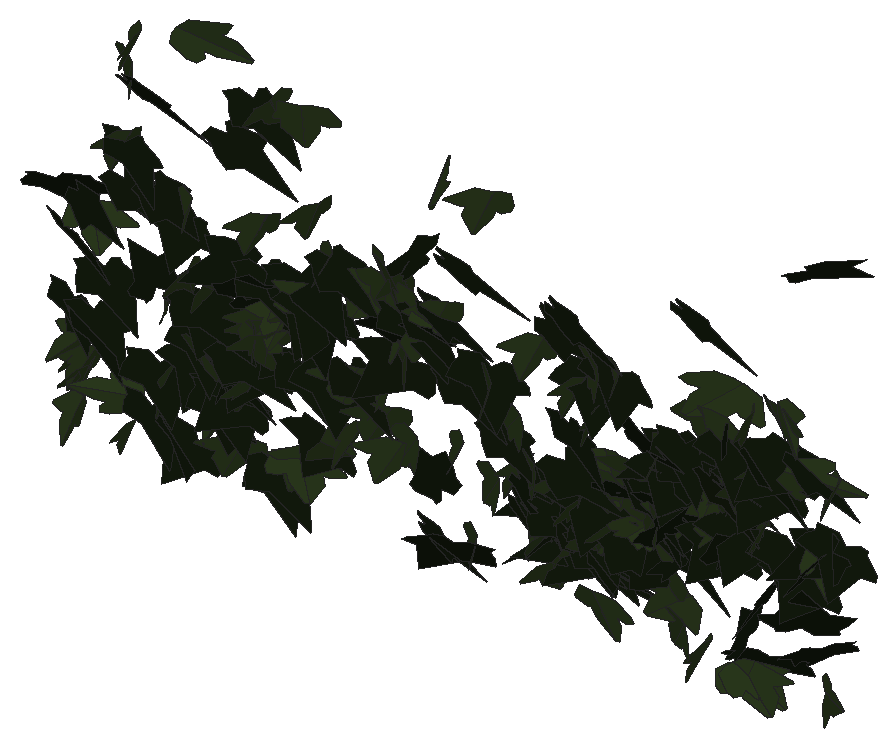
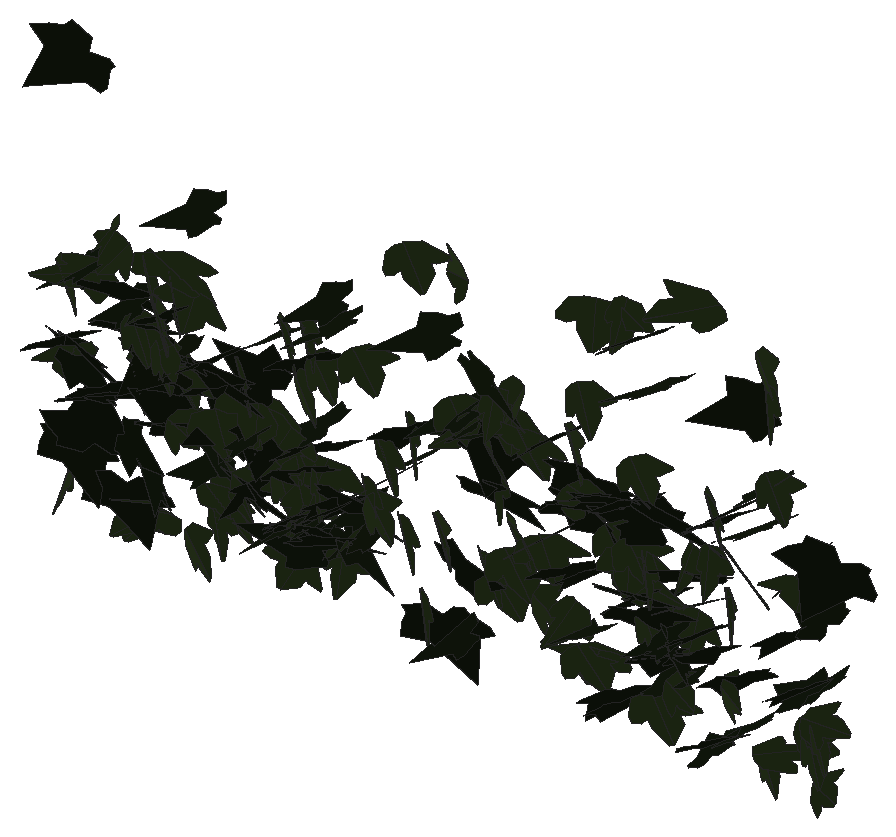
# SketchUp Ruby script. Lengths in millimetres.
U = 1.mm
M = Sketchup.active_model
def pt(a) = Geom::Point3d.new(a.map { |v| v * U })
def face(e, loops, mat)
  f = e.add_face(loops[0].map { |a| pt(a) })
  loops[1..].each { |l| e.add_face(l.map { |a| pt(a) }).erase! }
  f.material = f.back_material = mat if mat
  f
end
# faces: each face lists its corners as indices into pts; further lists are holes
def faces(e, pts, list, mat = nil) = list.each { |f| face(e, (f[0].is_a?(Array) ? f : [f]).map { |l| l.map { |i| pts[i] } }, mat) }
# xy, xz, yz: faces in a plane at the given z, y or x. An outline is a flat list of corners, or four numbers for a rectangle; further outlines are holes
def ring(l) = l.size == 4 ? [[l[0], l[1]], [l[2], l[1]], [l[2], l[3]], [l[0], l[3]]] : l.each_slice(2).to_a
def flat(e, list, mat, &to3) = list.each { |f| face(e, (f[0].is_a?(Array) ? f : [f]).map { |l| ring(l).map { |u, v| to3.(u, v) } }, mat) }
def xy(e, z, list, mat = nil) = flat(e, list, mat) { |x, y| [x, y, z] }
def xz(e, y, list, mat = nil) = flat(e, list, mat) { |x, z| [x, y, z] }
def yz(e, x, list, mat = nil) = flat(e, list, mat) { |y, z| [x, y, z] }
def lines(e, pts, list) = list.each { |a, b| e.add_line(pt(pts[a]), pt(pts[b])) }
# prism: a flat outline (further loops are holes) pulled along v
def prism(e, loops, v, mat = nil)
  f = face(e, loops, mat); d = Geom::Vector3d.new(v.map { |x| x * U })
  f.pushpull(f.normal.samedirection?(d) ? d.length : -d.length)
end
def box(e, o, s, mat = nil) = prism(e, [[o, [o[0] + s[0], o[1], o[2]], [o[0] + s[0], o[1] + s[1], o[2]], [o[0], o[1] + s[1], o[2]]]], [0, 0, s[2]], mat)
def at(x, y, z, deg = 0) = Geom::Transformation.translation(pt([x, y, z])) * Geom::Transformation.rotation(ORIGIN, Z_AXIS, deg.degrees)
def axes(o, x, y, z) = Geom::Transformation.new([*x, 0, *y, 0, *z, 0, *pt(o).to_a, 1])
def part(name) = M.definitions.add(name)
# library, detail: a bought-in or finely detailed component or shape, given as its bounding box
def library(name, o, s) = part(name).tap { |d| box(d.entities, o, s) }
def detail(e, o, s) = box(e.add_group.entities, o, s)
def put(e, d, t, mat = nil) = e.add_instance(d, t).tap { |i| i.material = mat if mat }
def group(e, t, mat = nil) = e.add_group.tap { |g| g.transformation = t; g.material = mat if mat }.entities
root = M.entities
M.materials.add("efeu1").color = [18, 25, 13]
M.materials.add("efeu2").color = [43, 57, 29]
c1 = part("ivyleaf_9")
p = [[39.1,54.8,31.7],[34.5,51.8,30.2],[-5.3,25.2,17.3],[-17.9,28.3,20.9],[-21.6,21.7,17],[-20.2,4.3,5.3],
  [-22.9,-0.3,2.5],[-17.1,-4,-0.6],[-2,-2.1,-1.2],[-0.7,-15.4,-10.1],[16.6,-22.3,-16.7],[21.1,-15.1,-12.5],
  [32.7,-10.7,-11],[46.1,-1.8,-6.6],[30.8,11.2,3.8]]
faces(c1.entities,p,[[0,1,2,3,4,5,6,7,8,9,10,11,12,13,14]],"efeu1")
c2 = part("ivyleaf_10")
p = [[0,12.8,-0.8],[-1.5,51.3,-10.9],[-4.9,51,-11.6],[-13.6,26.5,-7.3],[-13.2,15.9,-4.6],[-21.1,19.3,-7.2],
  [-29.5,16.3,-8.3],[-29.2,8.3,-6.2],[-19.7,-9.8,0.5],[-7.6,-13,4],[1,-12.2,5.8],[-0.4,51.1,-11.1],
  [-1.5,51.1,-10.9],[1,-12.4,5.9],[16.9,-12.4,3.5],[35.1,9.1,-5.1],[35,12.9,-6.1],[20.5,16.4,-4.9],
  [15.8,15,-3.8],[15.3,27.6,-7.1],[12.8,31.3,-7.8]]
faces(c2.entities,p,[[0,1,2,3,4,5,6,7,8,9,10],[11,12,0,13,14,15,16,17,18,19,20]],"efeu2")
put(root,c1,axes([2909.4,930.7,1858.6],[0.80138,-0.79258,-0.01396],[-0.02047,0.01009,-0.89748],[1.50854,0.42118,-0.00476]))
put(root,c1,axes([2143.2,933.4,1731.2],[-0.36983,-0.83025,-0.16051],[0.06105,0.15734,-0.85268],[1.60824,-0.1969,-0.00454]))
put(root,c1,axes([2156,908.4,1846.5],[-0.13639,0.4951,0.78388],[-0.38543,0.75888,-0.49782],[-1.72193,-0.20908,0.04934]))
put(root,c1,axes([2701.6,923.8,1996.9],[1.22093,-0.62842,-0.20152],[-0.109,0.22697,-0.89009],[1.25125,0.63296,0.1191]))
put(root,c1,axes([2747.7,937.1,1774.9],[-0.90081,-0.7438,0.00341],[-0.01004,-0.00068,-0.88162],[1.41559,-0.47333,-0.00408]))
put(root,c2,axes([2666.3,932.6,1941.3],[-0.66779,-0.78909,0.29764],[0.01925,-0.32629,-0.85311],[1.60496,-0.32441,0.13407]))
put(root,c1,axes([2267.2,916.4,1866.7],[0.4535,-0.06865,0.85647],[1.60668,0.18414,-0.22011],[-0.30437,0.86972,0.11421]))
put(root,c1,axes([2043.4,937.4,1745.9],[0.36348,-0.80234,0.30186],[0.21819,-0.28258,-0.82362],[1.61686,0.21851,0.04329]))
put(root,c2,axes([2309.2,917,2120.4],[-0.45151,-0.75455,-0.51758],[0.27982,0.49632,-0.79094],[1.71882,-0.27901,-0.0072]))
put(root,c1,axes([2255.4,923.3,1792.4],[0.4278,-0.6736,-0.50792],[0.182,0.54259,-0.67727],[1.59526,0.11874,0.21347]))
put(root,c1,axes([2503.9,931.8,1918.7],[0.6009,-0.84954,-0.04702],[0.07782,0.06525,-0.90426],[1.61744,0.31248,0.06097]))
put(root,c1,axes([2250.8,943,1722.3],[-1.09629,-0.52426,0.42323],[-0.25126,-0.4582,-0.74726],[1.25746,-0.54862,0.21967]))
put(root,c2,axes([2872.1,917.9,1669.4],[0.99405,-0.52607,-0.47161],[-0.15801,0.53672,-0.69065],[1.33533,0.45513,0.26935]))
put(root,c2,axes([2022.3,939.5,1637.2],[-0.10316,-0.63522,0.62819],[0.45465,-0.61674,-0.60302],[1.63837,0.13115,0.20689]))
put(root,c2,axes([2722.9,931.1,1913.7],[-0.16016,-0.88315,0.16431],[0.02444,-0.16619,-0.88671],[1.70948,-0.08036,0.02807]))
put(root,c1,axes([2127.9,938.4,1670.3],[0.03405,-0.85159,0.1942],[0.09251,-0.19296,-0.85067],[1.65978,0.02823,0.04343]))
put(root,c1,axes([2553.4,922.1,2006.6],[1.44064,-0.53989,-0.11564],[0.11771,0.27791,-0.89262],[1.0442,0.71353,0.26017]))
put(root,c1,axes([2170,941.6,1917.7],[-0.56197,-0.79681,0.27658],[-0.09246,-0.27649,-0.84841],[1.60259,-0.29537,0.04804]))
put(root,c1,axes([2686.8,925.7,1713.1],[-0.77621,0.68802,-0.30967],[0.24728,-0.28272,-0.79924],[-1.41451,-0.42697,0.03022]))
put(root,c1,axes([2492.9,937.6,1909.7],[-0.19363,-0.89325,0.00332],[0.6064,-0.03941,-0.83975],[1.58822,-0.09385,0.32103]))
put(root,c2,axes([2747.6,919.2,1734.6],[-0.66331,-0.67984,-0.44514],[0.39491,0.39384,-0.76396],[1.49528,-0.40559,0.0043]))
put(root,c2,axes([2296.2,924.1,1821.2],[-0.83165,-0.74668,-0.15234],[0.10766,0.14334,-0.86483],[1.44635,-0.44001,-0.02322]))
put(root,c1,axes([2694.6,926,1751.5],[0.13518,-0.72276,-0.49697],[0.06829,0.50057,-0.72287],[1.66795,0.03808,0.06987]))
put(root,c1,axes([3014.2,938.6,1913.5],[-1.56511,-0.36882,0.08779],[-0.06886,-0.13238,-0.89508],[0.71826,-0.81636,0.10548]))
put(root,c2,axes([2959.5,922.8,1639.8],[1.267,0.44384,0.35574],[0.53951,0.21589,-0.79985],[-0.93854,0.72327,0.02045]))
put(root,c2,axes([2269.5,928,1755.5],[-0.18091,-0.87217,-0.01301],[0.0017,0.01299,-0.87734],[1.6601,-0.09506,-0.00052]))
put(root,c1,axes([2207,930.3,1834.1],[-0.0734,-0.75829,-0.43226],[0.70025,0.37823,-0.69635],[1.50639,-0.21277,0.30264]))
put(root,c2,axes([2109.7,928.9,2128.3],[0.40809,-0.89774,-0.02066],[-0.00191,0.021,-0.92299],[1.70904,0.21439,0.0039]))
put(root,c2,axes([2695.2,920.7,1682.6],[-0.56416,-0.76683,-0.36816],[0.1952,0.35481,-0.8216],[1.60711,-0.31229,-0.02945]))
put(root,c1,axes([2950.7,939.7,1806.1],[-0.92835,-0.73922,0.07842],[-0.05571,-0.07463,-0.8855],[1.41369,-0.48838,0.01661]))
put(root,c1,axes([2770.7,942.2,1936],[-0.37873,-0.81888,0.29676],[0.06274,-0.31127,-0.83681],[1.65649,-0.17544,0.09955]))
put(root,c2,axes([2340.9,926.4,1685.7],[1.41976,0.41479,0.1404],[0.24538,0.05701,-0.85346],[-0.79648,0.75694,-0.01266]))
put(root,c1,axes([2246,926.3,2053.1],[0.78076,-0.76261,-0.33412],[0.17649,0.41201,-0.82653],[1.57472,0.33193,0.25829]))
put(root,c2,axes([2750.6,918.6,1947],[0.80962,-0.58843,-0.54919],[-0.23291,0.56667,-0.70195],[1.51407,0.40182,0.18569]))
put(root,c1,axes([2559.2,929.8,1865.2],[0.51469,-0.83253,-0.26467],[0.019,0.27999,-0.87051],[1.6625,0.25454,0.09189]))
put(root,c1,axes([2714.9,924.2,1814.2],[0.52598,-0.69901,-0.55122],[0.25405,0.60319,-0.69798],[1.67508,0.12801,0.27895]))
put(root,c1,axes([2850.7,908.1,1790.6],[-0.16075,0.36952,-0.82506],[-0.3573,0.80342,0.37904],[1.68304,0.20585,0.00167]))
put(root,c2,axes([2354.5,937.7,1885.2],[-0.82762,-0.4296,0.66141],[-0.64951,-0.57841,-0.60007],[1.3532,-0.54037,0.11649]))
put(root,c1,axes([3035.3,925.3,1929.4],[1.00991,-0.66287,-0.33758],[-0.18304,0.35005,-0.83854],[1.40387,0.52249,0.13352]))
put(root,c1,axes([2113.7,926.1,2070.3],[1.58521,-0.35872,0.14303],[0.24879,-0.05806,-0.90688],[0.6916,0.84311,-0.0016]))
put(root,c2,axes([2755.6,926.8,1657.6],[-1.45213,0.31812,-0.17894],[0.26229,-0.13286,-0.82385],[-0.64324,-0.77235,0.06802]))
put(root,c2,axes([2209.7,923.6,1775.3],[-1.48837,0.35112,0.08435],[-0.14945,0.03103,-0.85723],[-0.67081,-0.78596,0.00384]))
put(root,c1,axes([2237.4,935.1,1727.4],[-0.41639,-0.82495,-0.24624],[0.16874,0.23112,-0.85309],[1.62977,-0.2347,0.02541]))
put(root,c1,axes([2983.2,941.7,1876.2],[-1.30263,-0.58294,0.0227],[0.18862,-0.15067,-0.88107],[1.09416,-0.66804,0.1789]))
put(root,c2,axes([2867.7,925.6,1699],[1.32937,-0.30919,-0.4814],[-0.77172,0.26845,-0.76076],[0.76821,0.80472,0.06882]))
put(root,c1,axes([2276.3,932.1,2105.3],[0.27047,-0.86458,-0.27161],[0.16946,0.28692,-0.86673],[1.71641,0.10791,0.12837]))
put(root,c2,axes([2830.2,921.3,1791],[0.86804,-0.62,-0.44837],[-0.1241,0.4886,-0.74194],[1.45091,0.41272,0.20479]))
put(root,c2,axes([2603.8,919,1873.5],[0.58707,-0.76378,-0.61823],[-0.1577,0.62545,-0.81405],[1.86349,0.29355,0.12587]))
put(root,c1,axes([2012.9,941.7,1847.6],[0.3961,-0.66904,0.55304],[0.4288,-0.50759,-0.69884],[1.59541,0.30253,0.05052]))
put(root,c2,axes([2040.7,937.9,1706.9],[-0.2349,-0.76625,0.4123],[0.06756,-0.42052,-0.77089],[1.65466,-0.09161,0.09001]))
put(root,c2,axes([2720.9,925.6,1783.2],[-1.54855,-0.32982,-0.16392],[0.29727,0.05098,-0.87789],[0.63481,-0.82843,0.01124]))
put(root,c1,axes([2363.9,946.7,1708.3],[-0.78177,-0.60773,0.49349],[0.00071,-0.55744,-0.68619],[1.48993,-0.31861,0.25926]))
put(root,c1,axes([2805.4,920.5,1810.1],[1.29284,0.37606,-0.39581],[-0.70484,-0.14687,-0.77512],[-0.7635,0.77236,0.04533]))
put(root,c2,axes([2772.5,930,1752.5],[-0.17268,-0.85028,-0.01671],[0.00166,0.01671,-0.85511],[1.61857,-0.09073,-0.0009]))
put(root,c1,axes([2716.3,935.4,1727.3],[0.50332,-0.84439,-0.0439],[-0.03054,0.04097,-0.88483],[1.60893,0.26493,-0.00307]))
put(root,c2,axes([2726,923.5,1770.5],[-0.08377,-0.80556,-0.36166],[0.05612,0.36057,-0.80672],[1.67963,-0.05222,0.00892]))
put(root,c1,axes([2554.1,925,1657.2],[0.60631,0.61112,-0.55909],[-0.65256,-0.44798,-0.68505],[-1.43498,0.46193,0.0753]))
put(root,c2,axes([2596.1,933.9,2096.5],[-0.89565,-0.75334,0.21424],[-0.01311,-0.24595,-0.87997],[1.49056,-0.45483,0.12099]))
put(root,c1,axes([2363.7,942.7,1877.3],[-0.82308,-0.77497,0.13157],[-0.06355,-0.13192,-0.88679],[1.49467,-0.43236,0.03475]))
put(root,c2,axes([2359.7,929.2,2003.6],[-0.39285,-0.8997,-0.06173],[0.0093,0.06221,-0.92303],[1.71631,-0.20627,-0.00913]))
put(root,c2,axes([3011.8,927.5,1977.9],[-0.23118,0.88578,-0.09809],[0.01783,-0.09773,-0.89406],[-1.69602,-0.12177,0.00397]))
put(root,c1,axes([2289.6,932.8,1897.5],[0.06645,-0.84123,-0.33092],[0.11707,0.33261,-0.83904],[1.71646,0.00988,0.07004]))
put(root,c1,axes([2935.6,941.8,1904.6],[-0.48997,-0.84777,0.09368],[-0.02279,-0.09425,-0.88586],[1.62314,-0.25724,0.01584]))
put(root,c1,axes([2266.9,933.5,1896],[-1.6209,0.1504,0.18177],[-0.35197,-0.00282,-0.86417],[-0.27879,-0.87085,0.03419]))
put(root,c1,axes([2649.2,929.9,1762.8],[1.00563,-0.68049,-0.18562],[-0.16357,0.16808,-0.86085],[1.33241,0.53423,0.03441]))
put(root,c1,axes([2039.4,924.9,1911.3],[0.77836,-0.59364,-0.51117],[-0.50905,0.43617,-0.72054],[1.40136,0.48817,0.02218]))
put(root,c2,axes([2675.8,912,1714],[-0.06921,-0.1733,-0.89781],[0.33355,0.88054,-0.17706],[1.70798,-0.17898,-0.0018]))
put(root,c2,axes([2454.8,925.6,1970.3],[-0.88293,0.76914,-0.00582],[0.00547,-0.00506,-0.89822],[-1.46385,-0.46393,0.00015]))
put(root,c1,axes([2596,939.1,1882.7],[-0.45632,-0.85714,-0.10271],[0.04066,0.10067,-0.89002],[1.64248,-0.24063,-0.0065]))
put(root,c1,axes([2969.3,933.6,1902.3],[0.90871,-0.77371,-0.06069],[-0.0604,0.05174,-0.90917],[1.47581,0.47852,0.00016]))
put(root,c1,axes([2481.1,919.9,1904],[1.26064,0.53861,-0.27147],[-0.46438,-0.12946,-0.8522],[-1.0498,0.70405,0.05098]))
put(root,c1,axes([2351.3,937.1,1866.1],[-0.95766,-0.15655,-0.70433],[1.35564,0.02913,-0.51535],[0.21895,-0.86512,0.1101]))
put(root,c1,axes([3069.9,932.9,1823.1],[-1.59614,0.2784,-0.06454],[0.11299,-0.026,-0.88364],[-0.53203,-0.84074,0.00596]))
put(root,c1,axes([2385.5,930.4,1946.5],[0.4956,-0.79471,-0.38438],[-0.04016,0.39504,-0.83104],[1.67965,0.24394,0.09355]))
put(root,c1,axes([3059.3,933.9,1812.7],[-0.62235,0.59599,-0.5634],[0.48888,-0.50159,-0.67969],[-1.48235,-0.41565,0.01238]))
put(root,c1,axes([2015.2,944.1,1763.8],[0.10234,-0.80925,0.34041],[0.01368,-0.34063,-0.81091],[1.67083,0.05236,-0.01421]))
put(root,c1,axes([2222.6,946.5,1697.2],[-0.32614,-0.69715,0.48712],[0.21817,-0.51131,-0.69145],[1.60385,-0.07221,0.19311]))
put(root,c1,axes([2782.8,942.6,1871.4],[0.51669,-0.43402,0.79329],[0.71368,-0.69966,-0.51113],[1.56604,0.46205,-0.0288]))
put(root,c2,axes([2284.7,935.3,1841.7],[-0.67203,-0.7704,0.22773],[-0.08917,-0.22858,-0.84594],[1.52634,-0.35255,0.05085]))
put(root,c2,axes([2959.1,929.9,1953.9],[0.34956,-0.89419,-0.13502],[0.10629,0.14873,-0.90901],[1.71784,0.17275,0.08372]))
put(root,c1,axes([2870.2,926.7,1753.7],[-0.99186,0.71131,-0.10396],[0.13554,-0.07669,-0.88171],[-1.36142,-0.52586,-0.01204]))
put(root,c2,axes([2309.1,940.4,1854.6],[-0.69625,-0.70571,0.40923],[0.19495,-0.48469,-0.74425],[1.5403,-0.25765,0.27918]))
put(root,c2,axes([2771.8,928.9,1939.7],[0.69799,-0.81694,-0.21878],[-0.05025,0.22729,-0.89297],[1.60881,0.36153,0.06703]))
put(root,c1,axes([2851.7,944.2,1844],[-0.89488,-0.7567,0.0819],[0.05324,-0.11339,-0.88699],[1.44759,-0.46361,0.08325]))
put(root,c2,axes([2349.7,938,1687.2],[-0.88657,-0.6684,0.35346],[-0.15331,-0.36892,-0.80381],[1.43083,-0.45369,0.13288]))
put(root,c2,axes([2960,922.4,1641.9],[0.85557,0.52465,0.53791],[0.63232,0.42344,-0.69066],[-1.28269,0.55869,0.01832]))
put(root,c2,axes([3074.6,932.9,1907.2],[0.5494,-0.86911,-0.03695],[0.03219,0.04453,-0.9153],[1.65527,0.2876,0.03006]))
put(root,c1,axes([3027.9,936.7,1716.6],[1.38149,0.26863,0.52476],[-0.94813,-0.16555,0.77385],[0.5999,-0.88026,0.0146]))
put(root,c1,axes([2339.4,935.3,1909],[-0.61989,-0.45171,-0.70705],[1.22047,0.35507,-0.52225],[1.02972,-0.69277,0.19335]))
put(root,c2,axes([2147.8,942.8,1714.4],[0.38581,-0.66288,0.53641],[0.43104,-0.48971,-0.69076],[1.56463,0.29836,0.05803]))
put(root,c1,axes([2703.2,941.1,1848.1],[0.50053,-0.84001,0.1609],[0.07772,-0.15581,-0.88019],[1.62592,0.26604,-0.00746]))
put(root,c2,axes([2103.1,932.5,1644.1],[0.08856,-0.83337,-0.04496],[0.02224,0.04568,-0.83454],[1.58821,0.04583,0.01419]))
put(root,c1,axes([3033,947.1,1772.6],[-0.95688,-0.65718,0.26594],[-0.06454,-0.30336,-0.81377],[1.34773,-0.48112,0.14984]))
put(root,c2,axes([2461.4,930.4,1942.9],[-1.65897,0.19635,0.09667],[-0.24212,-0.13155,-0.8799],[-0.33893,-0.86709,0.15539]))
put(root,c1,axes([2614.8,934.1,1815.8],[0.47759,-0.8063,-0.26613],[-0.03176,0.27278,-0.84216],[1.61567,0.24371,0.06212]))
put(root,c2,axes([2341.6,930.5,2115.6],[-1.48048,-0.48788,-0.031],[0.08305,-0.01127,-0.91764],[0.92668,-0.77842,0.03272]))
put(root,c1,axes([2094,942,1985.4],[0.18452,-0.88731,0.07237],[0.02041,-0.07163,-0.89259],[1.69421,0.0975,0.00287]))
put(root,c2,axes([2804.7,938.9,1757.1],[0.78708,0.45844,-0.60027],[-0.91223,-0.36961,-0.6125],[-1.11096,0.62828,0.07767]))
put(root,c2,axes([3036.9,923,1913.5],[-0.50836,-0.16322,-0.85574],[1.50202,0.33366,-0.30999],[0.70205,-0.83205,0.04356]))
put(root,c1,axes([3078.9,946.4,1826.1],[-0.65041,-0.79021,0.20626],[-0.07931,-0.20643,-0.85989],[1.55228,-0.34164,0.04249]))
put(root,c2,axes([2780.2,929,1801.5],[-1.45672,0.19796,0.42981],[-0.84965,-0.03105,-0.78071],[-0.29863,-0.87728,0.12462]))
put(root,c2,axes([2898.4,932,1933.2],[-1.64281,0.17521,-0.08906],[0.10143,-0.17745,-0.86567],[-0.36004,-0.84943,0.16247]))
put(root,c1,axes([2339.2,937.7,1796.3],[0.09733,-0.86786,-0.22976],[0.07028,0.23197,-0.86799],[1.70717,0.03993,0.04883]))
put(root,c1,axes([2180.6,947.8,1641.5],[-0.82843,-0.6341,0.34252],[-0.21528,-0.33508,-0.76407],[1.35463,-0.44104,0.08805]))
put(root,c1,axes([2708.5,937.3,1762.5],[-1.62926,0.07646,0.18632],[-0.35471,0.00756,-0.85943],[-0.14525,-0.87607,0.00884]))
put(root,c2,axes([2579.2,927.9,1670.2],[0.63774,-0.71241,-0.32832],[0.00526,0.35809,-0.77419],[1.49292,0.30307,0.14298]))
put(root,c2,axes([2297.2,930.3,1801.9],[-0.12904,-0.01497,0.88164],[-1.6756,-0.04782,-0.06852],[0.09293,-0.88295,-0.01123]))
put(root,c2,axes([2024.8,947.5,1722.4],[-0.18523,-0.42905,0.75789],[-0.04277,-0.76111,-0.43377],[1.65696,-0.06761,0.07353]))
put(root,c2,axes([2607.7,926.6,1752.3],[0.83684,-0.68279,-0.43084],[-0.16965,0.44654,-0.79864],[1.52717,0.42375,0.14737]))
put(root,c2,axes([2404.1,943.7,1736.4],[0.11032,-0.74159,0.49205],[0.14471,-0.48717,-0.74318],[1.68762,0.09025,0.03156]))
put(root,c2,axes([2374,929.7,1945.9],[0.42207,-0.84703,-0.28223],[-0.08251,0.28025,-0.87514],[1.69719,0.22427,0.02764]))
put(root,c1,axes([2923.4,947.4,1776.6],[-1.3141,-0.50333,0.18217],[-0.02029,-0.28433,-0.82602],[1.01855,-0.65505,0.21857]))
put(root,c1,axes([2356.5,945.3,1872.3],[-1.09054,-0.68403,0.03057],[0.05223,-0.06278,-0.89021],[1.3021,-0.57038,0.06132]))
put(root,c1,axes([2738.3,944.3,1920],[-0.58818,-0.83537,0.01129],[0.00024,-0.01208,-0.8907],[1.59002,-0.30902,0.00431]))
put(root,c2,axes([2741.4,936.9,1883.6],[0.41414,-0.87161,0.09066],[0.08772,-0.0819,-0.89803],[1.6655,0.22105,0.02475]))
put(root,c1,axes([2687.9,925.9,1978.5],[1.11091,-0.50997,-0.4535],[-0.23377,0.5085,-0.72992],[1.27762,0.53647,0.26077]))
put(root,c2,axes([2476.8,938.9,1895.4],[0.81879,-0.77724,0.17532],[0.15059,-0.15658,-0.88834],[1.50892,0.43738,-0.00648]))
put(root,c1,axes([2970.2,914.9,1694.7],[-0.60436,0.22971,-0.89619],[-1.32211,0.56659,0.39137],[1.16291,0.76353,-0.0208]))
put(root,c1,axes([2193.2,947.2,1747.8],[-0.69019,-0.7536,0.205],[-0.15741,-0.18769,-0.83629],[1.47801,-0.3719,0.00666]))
put(root,c2,axes([2832.1,928.3,1868.6],[0.46629,-0.76909,-0.39565],[-0.15672,0.38861,-0.8064],[1.63859,0.25603,0.03547]))
put(root,c2,axes([2198.8,920.6,2164.6],[0.73658,0.19598,0.82773],[0.90895,0.70244,-0.38963],[-1.33963,0.58437,0.19075]))
put(root,c1,axes([2483.1,941.6,1850.8],[-1.68287,-0.15992,-0.0197],[0.0401,-0.00578,-0.89853],[0.30404,-0.88443,0.00944]))
put(root,c2,axes([2534.2,921.5,2081.9],[0.65247,-0.52953,0.67862],[-0.5407,0.61992,0.62725],[-1.54641,-0.44017,0.06701]))
put(root,c2,axes([2184.7,926.3,1862.7],[-0.18925,-0.77324,-0.46271],[0.1446,0.45667,-0.77947],[1.70889,-0.12427,0.01472]))
put(root,c2,axes([2973.4,934,1819.7],[0.44374,-0.83809,-0.10634],[0.05389,0.118,-0.86795],[1.60693,0.22747,0.05847]))
put(root,c2,axes([2857.7,925.7,1727.3],[-0.83566,0.34645,0.68714],[-1.26001,0.23321,-0.54063],[-0.74657,-0.78139,0.1433]))
put(root,c1,axes([2870.8,933.2,2051.3],[1.25791,-0.63081,-0.07012],[0.11514,0.1634,-0.89963],[1.20246,0.64426,0.1595]))
put(root,c1,axes([2927.7,920.9,1773],[0.01873,-0.18546,0.87666],[1.21982,0.61414,0.12273],[-1.19179,0.62567,0.13939]))
put(root,c2,axes([2465.5,940.2,1736.6],[-0.97686,-0.62942,0.32203],[-0.16458,-0.33906,-0.80055],[1.33549,-0.50218,0.13689]))
put(root,c1,axes([2861.1,944.9,1878.3],[-0.15904,-0.87928,0.04149],[-0.01195,-0.04108,-0.88324],[1.67526,-0.08377,-0.00236]))
put(root,c1,axes([2740,935.6,1723.1],[0.34268,-0.78707,-0.35039],[0.05645,0.36341,-0.80108],[1.63871,0.15207,0.10087]))
put(root,c1,axes([2990,928,1668.7],[0.70214,0.61662,-0.44663],[-0.62687,-0.31821,-0.71138],[-1.30645,0.48408,0.1013]))
put(root,c2,axes([2809.2,931,1834.2],[-1.79618,-0.01712,0.07843],[-0.14922,-0.00235,-0.94392],[0.03284,-0.94702,0.00092]))
put(root,c1,axes([2404.4,938,1813.9],[0.38693,-0.84803,-0.23704],[-0.01855,0.24109,-0.87089],[1.67573,0.19848,0.04509]))
put(root,c2,axes([2380.8,921.1,1723.9],[-0.40472,-0.59928,-0.74567],[0.54049,0.68989,-0.63544],[1.7386,-0.35397,0.02396]))
put(root,c2,axes([3072,924.1,1652],[0.42654,-0.63918,-0.5683],[0.32212,0.60901,-0.61823],[1.5956,0.04792,0.27672]))
put(root,c2,axes([2510.2,918.4,1909.9],[-0.08743,-0.42333,-0.93647],[1.00073,0.79574,-0.38551],[1.68055,-0.49587,0.18084]))
put(root,c1,axes([2228,942.2,1746.2],[-0.96248,0.29814,-0.64144],[0.97404,-0.39007,-0.58481],[-0.92926,-0.71766,0.05139]))
put(root,c2,axes([2527,940,1932.4],[-0.69637,-0.79289,0.22799],[-0.00369,-0.24858,-0.8676],[1.57017,-0.35223,0.09907]))
put(root,c2,axes([2634.1,928.6,1840.6],[0.97752,-0.58172,-0.4366],[-0.26333,0.44658,-0.75779],[1.359,0.50497,0.16721]))
put(root,c1,axes([2297.7,941.7,1648.8],[-0.11026,-0.83191,-0.14877],[0.00206,0.14905,-0.83388],[1.60841,-0.05722,-0.00913]))
put(root,c2,axes([2554.6,931.7,1774.7],[0.49636,-0.79449,-0.28458],[-0.11436,0.27962,-0.83571],[1.60207,0.26611,0.02851]))
put(root,c1,axes([3056.3,915.9,2176.2],[1.13549,0.59328,0.51411],[0.61219,0.40429,-0.83984],[-1.36291,0.67588,0.05108]))
put(root,c1,axes([2741.6,945.4,1728],[-0.05145,-0.87017,0.04415],[0.0214,-0.04452,-0.8705],[1.65811,-0.02642,0.0126]))
put(root,c2,axes([2856.3,938.4,1800.8],[-1.19006,-0.61241,0.15654],[-0.03419,-0.20289,-0.86548],[1.20253,-0.61183,0.13031]))
put(root,c2,axes([2888.7,940.5,1641.4],[0.26769,-0.87751,0.16074],[0.04352,-0.15913,-0.88871],[1.69732,0.14248,-0.00256]))
put(root,c1,axes([2642.3,931,1737.9],[1.09724,-0.53226,-0.37239],[-0.37722,0.33003,-0.77856],[1.17736,0.60178,0.09761]))
put(root,c1,axes([2792.9,931.3,1743.5],[0.25933,-0.66652,-0.62668],[-0.14641,0.623,-0.67933],[1.735,0.1522,0.03634]))
put(root,c1,axes([2739.6,944.7,1707.9],[-1.51435,-0.29816,0.05171],[-0.08713,-0.02519,-0.84968],[0.56931,-0.79697,0.00751]))
put(root,c1,axes([2978,943.9,1740.5],[-0.64384,0.38007,-0.70218],[0.77581,-0.57352,-0.50682],[-1.30663,-0.5278,0.04508]))
put(root,c2,axes([3060.5,935.8,1814.6],[0.78938,0.7663,-0.07857],[-0.05013,-0.07508,-0.87126],[-1.46521,0.41541,-0.01252]))
put(root,c2,axes([2272.5,926.7,1823.6],[0.73378,-0.60356,-0.56134],[-0.13847,0.59238,-0.68691],[1.56259,0.33592,0.20273]))
put(root,c1,axes([2695.8,948.1,1749.2],[-0.1858,-0.87575,0.11259],[-0.01177,-0.11259,-0.88115],[1.68041,-0.09762,0.00628]))
put(root,c2,axes([2655.2,929.9,1784.5],[0.83717,-0.64748,-0.40782],[-0.08599,0.4476,-0.75937],[1.4538,0.39933,0.18992]))
put(root,c2,axes([2752.3,940.6,1823.9],[1.34766,-0.28038,0.42554],[0.79417,-0.09916,-0.7597],[0.55673,0.82016,0.05362]))
put(root,c2,axes([2934.3,936.4,1857.4],[-0.10947,-0.87897,-0.07927],[0.04312,0.07794,-0.88067],[1.67909,-0.05931,0.01745]))
put(root,c2,axes([2444,939.7,1809.8],[0.91875,-0.73974,0.02869],[0.03221,-0.02322,-0.88332],[1.40857,0.48304,0.00148]))
put(root,c1,axes([2721.9,949.7,1703],[-1.24848,-0.24274,0.48225],[-0.72724,-0.32739,-0.68456],[0.72592,-0.74546,0.14361]))
put(root,c1,axes([2300.8,939.2,1659.7],[-0.05877,-0.80519,-0.39924],[0.05208,0.39845,-0.80571],[1.70968,-0.03982,0.01082]))
put(root,c2,axes([2927.3,939.1,1972.4],[1.55638,0.15887,-0.54508],[-1.04152,-0.03404,-0.83094],[-0.28784,0.98219,0.05937]))
put(root,c1,axes([3059.4,928.9,1702.3],[0.24923,0.85091,-0.23638],[-0.13992,-0.22764,-0.86015],[-1.67495,0.14563,0.03668]))
put(root,c1,axes([2372.7,947.5,1790.9],[-0.50232,-0.84156,-0.04058],[0.0347,0.03681,-0.88195],[1.60314,-0.26449,0.00638]))
put(root,c1,axes([2535,925.3,1722.6],[-0.1603,0.107,0.87489],[-0.73419,0.78575,-0.13324],[-1.5083,-0.39385,-0.02813]))
put(root,c1,axes([2801,943,1803.4],[0.68741,-0.79465,-0.00055],[0.00013,0.00063,-0.87288],[1.51237,0.36119,0.00032]))
put(root,c1,axes([2836.7,930.1,1725.9],[-1.0517,0.53484,0.54174],[-0.81592,0.33455,-0.76759],[-1.19728,-0.6978,0.04722]))
put(root,c2,axes([2101.3,928.9,2090.9],[0.76494,-0.66154,-0.4994],[-0.04113,0.54646,-0.74127],[1.57697,0.33514,0.22291]))
put(root,c1,axes([2267.7,948.2,1774.9],[-1.20198,-0.61459,-0.02176],[0.02901,0.01553,-0.88124],[1.17006,-0.63174,-0.0005]))
put(root,c2,axes([2432.8,937.3,1928.3],[1.65875,-0.13694,-0.20885],[-0.36463,0.11975,-0.87803],[0.30491,0.8882,0.08618]))
put(root,c2,axes([2088.7,940.6,1992.2],[-0.36501,-0.87342,0.1034],[-0.00421,-0.10535,-0.894],[1.6739,-0.19072,0.0203]))
put(root,c1,axes([2061.7,941.5,1817.2],[0.03373,-0.83507,-0.3101],[0.01611,0.31031,-0.83514],[1.69527,0.01367,0.01411]))
put(root,c1,axes([2862,940.8,1850.1],[-1.63934,0.18451,0.04284],[-0.0698,0.03324,-0.88055],[-0.35368,-0.86178,-0.02479]))
put(root,c1,axes([2857.2,942.8,1747.3],[0.85392,-0.74076,0.03737],[0.03141,-0.03369,-0.86604],[1.41126,0.44896,-0.00334]))
put(root,c1,axes([2927.1,923.3,1907.2],[0.11004,-0.11447,0.88511],[0.24518,0.87875,0.10523],[-1.68079,0.12069,0.0733]))
put(root,c2,axes([2216.3,949.5,1699.2],[-0.10856,-0.70475,0.51976],[0.24018,-0.52204,-0.69399],[1.6492,0.02964,0.13528]))
put(root,c2,axes([2248,941.4,1665.1],[-1.04295,-0.65177,0.21333],[-0.18836,-0.19506,-0.85016],[1.29155,-0.55477,0.04828]))
put(root,c2,axes([2403.4,942.4,1806.7],[-1.15899,-0.6118,0.19593],[-0.04024,-0.25074,-0.84865],[1.22196,-0.58853,0.15788]))
put(root,c1,axes([2753.4,931,1711.3],[1.01681,-0.47664,-0.49908],[-0.39281,0.49191,-0.69074],[1.25332,0.54087,0.18841]))
put(root,c1,axes([2092.8,939.3,1938.5],[0.62083,-0.77871,-0.29159],[0.15456,0.34157,-0.82132],[1.57497,0.27344,0.19554]))
put(root,c2,axes([2932.6,940.7,1865.4],[-1.22248,0.37563,-0.49597],[0.74626,-0.30905,-0.74189],[-0.91933,-0.75037,0.05728]))
put(root,c2,axes([2289.3,936.7,1829.1],[-1.10285,-0.65111,-0.09346],[0.1013,0.07773,-0.87155],[1.24779,-0.58179,-0.01185]))
put(root,c2,axes([2903.8,941.2,1848.3],[1.45772,-0.47573,-0.00913],[0.00248,0.0194,-0.90149],[0.90558,0.76574,0.01717]))
put(root,c2,axes([2943,935.6,1907.1],[0.47171,-0.82408,-0.29428],[-0.1169,0.28872,-0.86024],[1.66129,0.25431,0.02303]))
put(root,c2,axes([2485.8,936.2,1755.1],[0.97344,-0.64356,-0.29086],[-0.18345,0.29215,-0.81593],[1.33153,0.51074,0.10022]))
put(root,c2,axes([2152.6,933.2,1823.1],[0.50929,-0.73751,-0.40182],[0.00494,0.42245,-0.77364],[1.59844,0.23368,0.13042]))
put(root,c1,axes([2285,952.3,1794.5],[-1.52924,-0.35056,0.01012],[0.17201,-0.23142,-0.84077],[0.64493,-0.76953,0.24824]))
put(root,c1,axes([2869.8,946.8,1864.3],[-1.63529,-0.01561,0.18594],[-0.34966,-0.08243,-0.85589],[0.0621,-0.87525,0.07729]))
put(root,c1,axes([2159.2,955.7,1639.5],[-0.11041,-0.67643,0.53877],[0.0159,-0.5404,-0.67757],[1.64576,-0.04016,0.04269]))
put(root,c1,axes([2044,945.1,1756.8],[0.08566,-0.84877,-0.2057],[0.08505,0.20794,-0.84824],[1.65997,0.03314,0.05408]))
put(root,c2,axes([2476.7,931.9,1860.5],[0.82806,-0.63287,-0.47452],[-0.09426,0.51871,-0.73722],[1.5025,0.38133,0.21527]))
put(root,c2,axes([2209.3,927.2,1855.9],[-0.03715,-0.57992,-0.6969],[0.24081,0.6885,-0.57647],[1.70861,-0.10965,0.06609]))
put(root,c2,axes([2034.6,938.1,1686.1],[-0.15676,-0.8522,-0.16457],[-0.00375,0.16549,-0.85599],[1.65187,-0.0805,-0.01756]))
put(root,c2,axes([2046,939.2,1885],[1.11964,0.65833,0.0137],[0.05909,-0.00938,-0.88239],[-1.25181,0.58838,-0.0294]))
put(root,c1,axes([2715.2,941.6,1692.6],[0.99093,-0.48003,0.49711],[0.99353,-0.13461,-0.67676],[0.86178,0.70717,0.20862]))
put(root,c2,axes([2447.9,943.3,1774.3],[-0.96176,-0.70939,0.2274],[-0.24063,-0.18913,-0.87095],[1.39721,-0.52087,0.00654]))
put(root,c1,axes([2189.4,951.6,1774.5],[-0.27726,-0.86073,0.08094],[0.00248,-0.0823,-0.87285],[1.64537,-0.14492,0.01495]))
put(root,c1,axes([2136.7,937.3,1945.9],[0.64373,-0.70391,-0.45854],[-0.09323,0.47694,-0.7683],[1.59614,0.31175,0.14005]))
put(root,c2,axes([2026.7,938.7,1706.5],[0.10737,-0.848,-0.17399],[0.00776,0.17461,-0.84973],[1.64751,0.05444,0.01534]))
put(root,c2,axes([2082.3,952.1,1664.2],[-0.02794,0.28991,0.81988],[-0.68906,-0.74759,0.25787],[1.50482,-0.33694,0.1333]))
put(root,c1,axes([2503.5,937.5,1992.3],[-1.00512,0.71989,-0.16553],[0.18307,-0.13473,-0.89283],[-1.39387,-0.5368,0.0021]))
put(root,c2,axes([2902,952.7,1784.3],[-0.1265,-0.66066,0.57596],[0.18491,-0.57961,-0.65363],[1.65781,0.01424,0.11685]))
put(root,c1,axes([3005.8,951.8,1794.6],[-0.64375,-0.8139,0.00539],[0.00127,-0.00611,-0.88138],[1.54905,-0.33823,0.00296]))
put(root,c1,axes([2926.9,931.8,1854.2],[1.66807,-0.01594,-0.19155],[-0.36003,0.08691,-0.8728],[0.06482,0.89292,0.08154]))
put(root,c2,axes([2172.3,940,1938],[0.78022,-0.79288,-0.14683],[0.01438,0.16849,-0.88873],[1.53461,0.40154,0.08298]))
put(root,c2,axes([2272.8,945.2,1949.9],[-0.53586,-0.81794,0.18961],[-0.01577,-0.19727,-0.86329],[1.59791,-0.27624,0.05506]))
put(root,c2,axes([2476.3,933.4,1958.7],[-0.30812,-0.78602,-0.44335],[0.24655,0.42553,-0.80171],[1.69973,-0.20421,0.03592]))
put(root,c1,axes([2512.9,935.4,1932.5],[1.25782,-0.51762,-0.33874],[-0.23724,0.3741,-0.81485],[1.15319,0.64155,0.20184]))
put(root,c1,axes([2197.4,956.3,1809.2],[-0.65767,-0.7508,0.27495],[0.01773,-0.30329,-0.81648],[1.52162,-0.32097,0.12835]))
put(root,c2,axes([2965.1,943.4,1882.7],[-0.31991,-0.88289,0.05335],[0.02369,-0.05667,-0.89846],[1.68321,-0.167,0.02279]))
put(root,c2,axes([2632.8,946.5,1775.8],[-0.03829,-0.85394,0.19368],[0.02804,-0.19403,-0.85397],[1.66627,-0.01636,0.01882]))
put(root,c1,axes([2006.4,928.8,1916.1],[1.43198,0.5911,-0.06795],[-0.10074,-0.04262,-0.95682],[-1.12789,0.75427,-0.00081]))
put(root,c1,axes([2512.5,937,1656.9],[1.26482,-0.46572,-0.27422],[-0.28193,0.26102,-0.8023],[0.98921,0.66987,0.12196]))
put(root,c2,axes([2990.5,940.6,1968],[-1.1229,0.63296,-0.23476],[0.32313,-0.16263,-0.86521],[-1.24355,-0.61382,-0.01284]))
put(root,c1,axes([2220.1,942.1,1759.3],[1.0422,-0.67579,-0.17608],[-0.13651,0.16815,-0.86842],[1.32208,0.55009,0.04914]))
